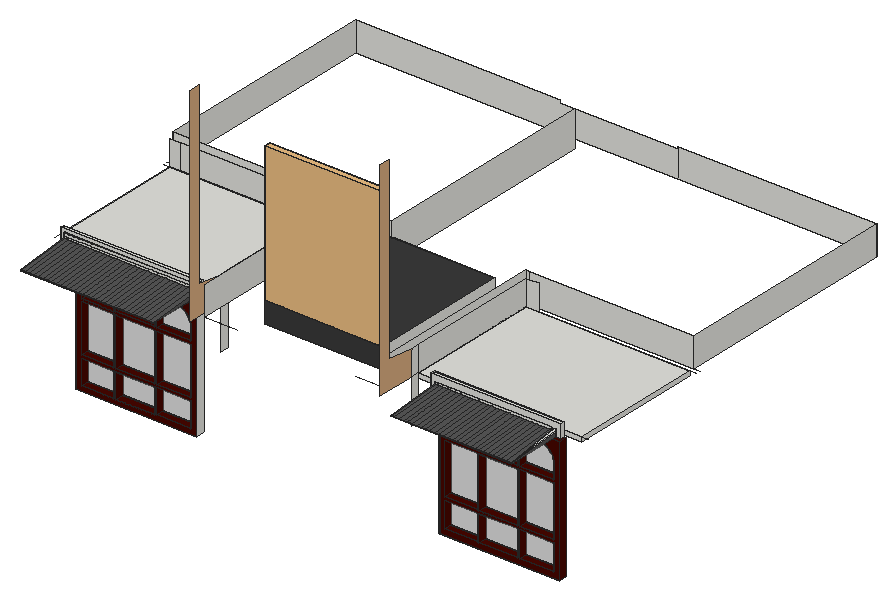
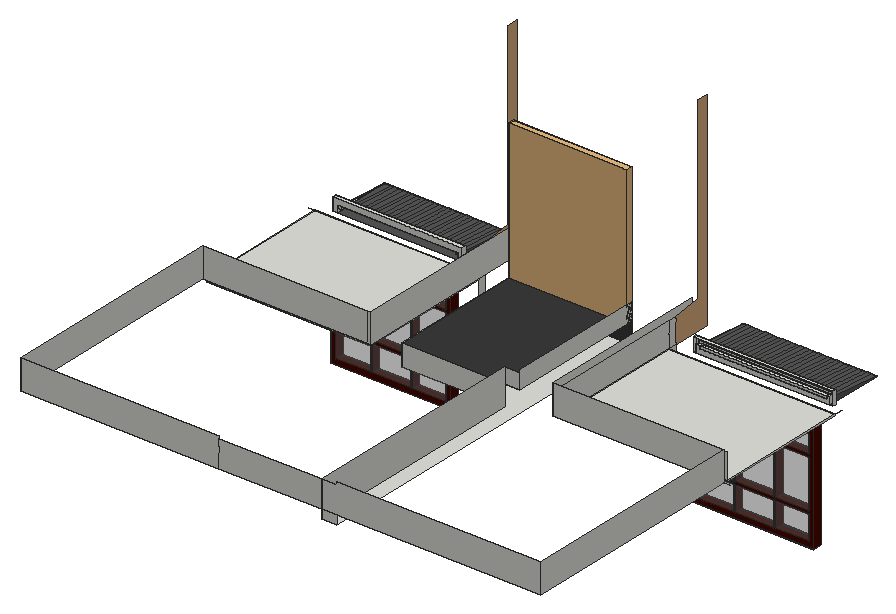
# SketchUp Ruby script. Lengths in inches.
U = 1.inch
M = Sketchup.active_model
def pt(a) = Geom::Point3d.new(a.map { |v| v * U })
def face(e, loops, mat)
  f = e.add_face(loops[0].map { |a| pt(a) })
  loops[1..].each { |l| e.add_face(l.map { |a| pt(a) }).erase! }
  f.material = f.back_material = mat if mat
  f
end
# faces: each face lists its corners as indices into pts; further lists are holes
def faces(e, pts, list, mat = nil) = list.each { |f| face(e, (f[0].is_a?(Array) ? f : [f]).map { |l| l.map { |i| pts[i] } }, mat) }
# xy, xz, yz: faces in a plane at the given z, y or x. An outline is a flat list of corners, or four numbers for a rectangle; further outlines are holes
def ring(l) = l.size == 4 ? [[l[0], l[1]], [l[2], l[1]], [l[2], l[3]], [l[0], l[3]]] : l.each_slice(2).to_a
def flat(e, list, mat, &to3) = list.each { |f| face(e, (f[0].is_a?(Array) ? f : [f]).map { |l| ring(l).map { |u, v| to3.(u, v) } }, mat) }
def xy(e, z, list, mat = nil) = flat(e, list, mat) { |x, y| [x, y, z] }
def xz(e, y, list, mat = nil) = flat(e, list, mat) { |x, z| [x, y, z] }
def yz(e, x, list, mat = nil) = flat(e, list, mat) { |y, z| [x, y, z] }
def lines(e, pts, list) = list.each { |a, b| e.add_line(pt(pts[a]), pt(pts[b])) }
# prism: a flat outline (further loops are holes) pulled along v
def prism(e, loops, v, mat = nil)
  f = face(e, loops, mat); d = Geom::Vector3d.new(v.map { |x| x * U })
  f.pushpull(f.normal.samedirection?(d) ? d.length : -d.length)
end
def box(e, o, s, mat = nil) = prism(e, [[o, [o[0] + s[0], o[1], o[2]], [o[0] + s[0], o[1] + s[1], o[2]], [o[0], o[1] + s[1], o[2]]]], [0, 0, s[2]], mat)
def at(x, y, z, deg = 0) = Geom::Transformation.translation(pt([x, y, z])) * Geom::Transformation.rotation(ORIGIN, Z_AXIS, deg.degrees)
def axes(o, x, y, z) = Geom::Transformation.new([*x, 0, *y, 0, *z, 0, *pt(o).to_a, 1])
def part(name) = M.definitions.add(name)
# library, detail: a bought-in or finely detailed component or shape, given as its bounding box
def library(name, o, s) = part(name).tap { |d| box(d.entities, o, s) }
def detail(e, o, s) = box(e.add_group.entities, o, s)
def put(e, d, t, mat = nil) = e.add_instance(d, t).tap { |i| i.material = mat if mat }
def group(e, t, mat = nil) = e.add_group.tap { |g| g.transformation = t; g.material = mat if mat }.entities
root = M.entities
M.materials.add("[Color C04]").color = [215, 171, 127]
M.materials.add("[Color C08]").color = [71, 7, 0]
M.materials.add("[Color M06]").color = [86, 86, 86]
M.materials.add("[Color M07]").color = [58, 58, 58]
M.materials.add("[Translucent Glass Gray]").color = [128, 128, 128]
M.materials["[Translucent Glass Gray]"].alpha = 0.5
c1 = part("Group\#1")
xy(c1.entities,0,[[0,0,133.1875,11.375]],"[Color C08]")
xy(c1.entities,6.44,[[6.44,0,42.59,11.375],[44.75,0,86.9,11.375],[89.0625,0,126.75,11.375]],"[Color C08]")
xy(c1.entities,37.85,[[6.44,0,42.59,11.375],[44.75,0,86.9,11.375],[89.0625,0,126.75,11.375]],"[Color C08]")
xy(c1.entities,40.75,[[6.44,0,42.59,11.375],[44.75,0,86.9,11.375],[89.0625,0,126.75,11.375]],"[Color C08]")
xy(c1.entities,101.6,[[6.44,0,42.59,11.375],[44.75,0,86.9,11.375],[89.0625,0,126.75,11.375]],"[Color C08]")
xy(c1.entities,104.5,[[6.44,0,42.59,11.375],[44.75,0,86.9,11.375],[89.0625,0,126.75,11.375]],"[Color C08]")
xy(c1.entities,140.62,[[24.51,0,42.59,11.375],[44.75,0,86.9,11.375],[89.0625,0,107.9,11.375]],"[Color C08]")
xy(c1.entities,147.0625,[[0,0,133.1875,11.375]],"[Color C08]")
xz(c1.entities,0,[[[0,0,133.1875,147.0625],[44.75,40.75,86.9,101.6],[89.0625,40.75,126.75,101.6],[6.44,40.75,42.59,101.6],[44.75,104.5,86.9,140.62],[44.75,6.44,86.9,37.85],[89.0625,104.5,89.0625,140.62,107.9,140.62,110.36,140.46,112.78,139.98,115.11,139.1875,117.33,138.1,119.375,136.73,121.23,135.1,122.85,133.25,124.22,131.2,125.3125,128.99,126.1,126.66,126.58,124.24,126.75,121.78,126.75,104.5],[6.44,104.5,6.44,127.03,6.65,127.83,7.8,130.52,9.36,133,11.29,135.21,13.53,137.09,16.03,138.61,18.75,139.72,21.59,140.39,24.51,140.62,42.59,140.62,42.59,104.5],[89.0625,6.44,126.75,37.85],[6.44,6.44,42.59,37.85]]],"[Color C08]")
xz(c1.entities,11.375,[[[0,0,133.1875,147.0625],[44.75,40.75,86.9,101.6],[89.0625,40.75,126.75,101.6],[6.44,40.75,42.59,101.6],[44.75,104.5,86.9,140.62],[44.75,6.44,86.9,37.85],[89.0625,104.5,126.75,104.5,126.75,121.78,126.58,124.24,126.1,126.66,125.3125,128.99,124.22,131.2,122.85,133.25,121.23,135.1,119.375,136.73,117.33,138.1,115.11,139.1875,112.78,139.98,110.36,140.46,107.9,140.62,89.0625,140.62],[6.44,104.5,42.59,104.5,42.59,140.62,24.51,140.62,21.59,140.39,18.75,139.72,16.03,138.61,13.53,137.09,11.29,135.21,9.36,133,7.8,130.52,6.65,127.83,6.44,127.03],[89.0625,6.44,126.75,37.85],[6.44,6.44,42.59,37.85]]],"[Color C08]")
xz(c1.entities,11.375,[[6.44,6.44,42.59,37.85],[44.75,6.44,86.9,37.85],[89.0625,6.44,126.75,37.85],[6.44,40.75,42.59,101.6],[44.75,40.75,86.9,101.6],
  [89.0625,40.75,126.75,101.6],[6.44,104.5,42.59,104.5,42.59,140.62,24.51,140.62,21.59,140.39,18.75,139.72,16.03,138.61,13.53,137.09,11.29,135.21,9.36,133,7.8,130.52,6.65,127.83,6.44,127.03],[44.75,104.5,86.9,140.62],[89.0625,104.5,126.75,104.5,126.75,121.78,126.58,124.24,126.1,126.66,125.3125,128.99,124.22,131.2,122.85,133.25,121.23,135.1,119.375,136.73,117.33,138.1,115.11,139.1875,112.78,139.98,110.36,140.46,107.9,140.62,89.0625,140.62]],"[Translucent Glass Gray]")
yz(c1.entities,0,[[0,0,11.375,147.0625]],"[Color C08]")
yz(c1.entities,6.44,[[0,6.44,11.375,37.85],[0,40.75,11.375,101.6],[0,104.5,11.375,127.03]],"[Color C08]")
yz(c1.entities,42.59,[[0,6.44,11.375,37.85],[0,40.75,11.375,101.6],[0,104.5,11.375,140.62]],"[Color C08]")
yz(c1.entities,44.75,[[0,6.44,11.375,37.85],[0,40.75,11.375,101.6],[0,104.5,11.375,140.62]],"[Color C08]")
yz(c1.entities,86.9,[[0,6.44,11.375,37.85],[0,40.75,11.375,101.6],[0,104.5,11.375,140.62]],"[Color C08]")
yz(c1.entities,89.0625,[[0,6.44,11.375,37.85],[0,40.75,11.375,101.6],[0,104.5,11.375,140.62]],"[Color C08]")
yz(c1.entities,126.75,[[0,6.44,11.375,37.85],[0,40.75,11.375,101.6],[0,104.5,11.375,121.78]],"[Color C08]")
yz(c1.entities,133.1875,[[0,0,11.375,147.0625]],"[Color C08]")
p = [[126.58,11.375,124.24],[126.75,11.375,121.78],[126.75,0,121.78],[126.58,0,124.24],[126.1,11.375,126.66],[126.1,0,126.66],
  [125.3125,11.375,128.99],[125.3125,0,128.99],[6.44,11.375,127.03],[6.65,11.375,127.83],[6.65,0,127.83],[6.44,0,127.03],
  [7.8,11.375,130.52],[7.8,0,130.52],[124.22,11.375,131.2],[124.22,0,131.2],[9.36,11.375,133],[9.36,0,133],
  [122.85,11.375,133.25],[122.85,0,133.25],[11.29,11.375,135.21],[11.29,0,135.21],[121.23,11.375,135.1],[121.23,0,135.1],
  [119.375,11.375,136.73],[119.375,0,136.73],[13.53,11.375,137.09],[13.53,0,137.09],[117.33,11.375,138.1],[117.33,0,138.1],
  [16.03,11.375,138.61],[16.03,0,138.61],[115.11,11.375,139.1875],[115.11,0,139.1875],[18.75,11.375,139.72],[18.75,0,139.72],
  [112.78,11.375,139.98],[112.78,0,139.98],[21.59,11.375,140.39],[21.59,0,140.39],[110.36,11.375,140.46],[110.36,0,140.46],
  [24.51,11.375,140.62],[24.51,0,140.62],[107.9,11.375,140.62],[107.9,0,140.62]]
faces(c1.entities,p,[[0,1,2,3],[4,0,3,5],[6,4,5,7],[8,9,10,11],[9,12,13,10],[14,6,7,15],[12,16,17,13],[18,14,15,19],
  [16,20,21,17],[22,18,19,23],[24,22,23,25],[20,26,27,21],[28,24,25,29],[26,30,31,27],[32,28,29,33],[30,34,35,31],
  [36,32,33,37],[34,38,39,35],[40,36,37,41],[38,42,43,39],[44,40,41,45]],"[Color C08]")
c2 = library("Group\#2",[0,0,0],[72,4.0625,96])
xy(root,60.79,[[546.77,627.4375,708.59,638.0625]])
xy(root,63.5625,[[57.38,626.0625,219.82,638.0625]])
xy(root,221.625,[[57.38,626.0625,219.82,638.0625]])
xy(root,224.25,[[303.29,636.875,303.29,1134.4375,323.73,1134.4375,323.73,826.22,462.79,826.22,462.79,636.875]])
xy(root,227.85,[[546.77,627.4375,708.59,638.0625]])
xy(root,231,[[509.3125,638.0625,730.375,820.1875]])
xy(root,235,[[28.375,638.0625,252.9375,820.1875]])
xy(root,237,[[40.76,621.9375,45.125,626.0625],[225.1875,621.9375,228.51,626.0625],[539.72,621.9375,545.41,627.4375],[708.06,621.9375,714.84,627.4375],[28.375,638.0625,252.9375,820.1875],
  [509.3125,638.0625,730.375,820.1875]])
xy(root,237,[[45.125,547.4375,225.1875,626.0625],[545.41,547.4375,708.06,627.4375]],"[Color M06]")
xy(root,243.26,[[545.41,621.9375,548.77,627.4375]])
xy(root,243.75,[[48.93,621.9375,219.99,626.0625]])
xy(root,244.125,[[219.99,620.875,219.99,621.9375,48.93,621.9375,55,621.9,64,621.84]])
xy(root,246.3125,[[545.41,621.9375,548.77,627.4375],[548.77,621.9375,702.25,627.4375],[702.25,621.9375,708.06,627.4375]])
xy(root,247.25,[[45.125,620.875,48.93,626.0625],[48.93,620.875,219.99,621.9375],[219.99,620.875,225.1875,626.0625],[48.93,621.9375,219.99,626.0625]])
xy(root,251,[[45.125,620.875,225.1875,621.9375]])
xy(root,252.9375,[[303.29,636.875,462.79,826.22]],"[Color M07]")
xy(root,254.125,[[539.72,621.9375,714.84,627.4375]])
xy(root,255.5,[[40.76,621.9375,228.51,626.0625]])
xz(root,547.4375,[[45.125,237,225.1875,237.93],[545.41,237,708.06,237.6875]])
xz(root,620.875,[[45.125,244.125,225.1875,247.25],[45.125,247.25,225.1875,251]])
xz(root,621.9375,[[40.76,237,45.125,237,45.125,251,225.1875,251,225.1875,237,228.51,237,228.51,255.5,40.76,255.5],[539.72,237,545.41,237,545.41,246.3125,708.06,246.3125,708.06,237,714.84,237,714.84,254.125,539.72,254.125],[548.77,243.26,702.25,246.3125],[48.93,243.75,219.99,244.125],[48.93,244.125,219.99,247.25]])
xz(root,626.0625,[[45.125,237,45.125,247.25,48.93,247.25,48.93,243.75,219.99,243.75,219.99,247.25,225.1875,247.25,225.1875,237],[48.93,243.75,219.99,247.25]])
xz(root,627.4375,[[539.72,237,539.72,254.125,714.84,254.125,714.84,237,708.06,237,708.06,246.3125,545.41,246.3125,545.41,237],[545.41,243.26,548.77,246.3125],[702.25,243.26,708.06,246.3125]])
xz(root,636.875,[[303.29,224.25,462.79,252.9375]],"[Color M07]")
xz(root,638.0625,[[509.3125,231,730.375,237],[28.375,235,252.9375,237]])
xz(root,820.1875,[[509.3125,231,526.3125,237],[526.3125,231,730.375,237],[28.375,235,42.875,237],[42.875,235,252.9375,237],[28.375,237,42.875,271.1875],
  [42.875,237,252.9375,271.1875],[509.3125,237,526.3125,271.1875]])
xz(root,826.1875,[[28.375,237,258.9375,276.1875],[509.3125,237,730.375,276.1875]])
xz(root,826.22,[[323.73,224.25,462.79,252.9375],[303.29,252.9375,323.73,273.1875]])
xz(root,1134.4375,[[303.29,224.25,323.73,237],[28.375,237,323.73,237,323.73,273.1875,303.29,273.1875,303.29,276.1875,28.375,276.1875],[323.73,237,462.79,273.1875],[462.79,237,730.375,276.1875]])
yz(root,28.375,[[638.0625,235,820.1875,237],[826.1875,237,1134.4375,276.1875]])
yz(root,40.76,[[621.9375,237,626.0625,255.5]])
yz(root,45.125,[[621.9375,237,626.0625,247.25],[620.875,247.25,621.9375,251]])
yz(root,45.125,[[547.4375,237,547.4375,237.93,620.875,244.125,620.875,247.25,621.9375,247.25,621.9375,237]],"[Color M06]")
yz(root,48.93,[[621.9375,243.75,626.0625,247.25]])
yz(root,57.38,[[626.0625,63.5625,638.0625,221.625]])
yz(root,219.82,[[626.0625,63.5625,638.0625,221.625]])
yz(root,219.99,[[621.9375,243.75,626.0625,247.25]])
yz(root,225.1875,[[621.9375,237,626.0625,247.25],[620.875,247.25,621.9375,251]])
yz(root,225.1875,[[547.4375,237,621.9375,237,621.9375,247.25,620.875,247.25,620.875,244.125,547.4375,237.93]],"[Color M06]")
yz(root,228.51,[[621.9375,237,626.0625,255.5]])
yz(root,252.9375,[[626.0625,177,638.0625,237],[638.0625,235,820.1875,237],[626.0625,237,638.0625,271.1875],[638.0625,237,820.1875,271.1875]])
yz(root,252.9375,[[573.625,237,573.625,516.1875,588.625,516.1875,588.625,275.59,626.0625,271.1875,626.0625,237]],"[Color C04]")
yz(root,258.9375,[[590.9375,237,826.1875,276.1875]])
yz(root,303.29,[[636.875,252.9375,826.22,276.1875]])
yz(root,323.73,[[826.22,224.25,1134.4375,273.1875]])
yz(root,462.79,[[636.875,224.25,826.22,237],[636.875,237,826.22,252.9375]])
yz(root,503.3125,[[590.9375,237,826.375,276.1875]])
yz(root,509.3125,[[627.4375,177,638.0625,237],[638.0625,231,820.1875,237],[627.4375,237,638.0625,271.1875],[638.0625,237,820.1875,271.1875]])
yz(root,509.3125,[[573.625,237,627.4375,237,627.4375,271.1875,588.625,275.59,588.625,516.1875,573.625,516.1875]],"[Color C04]")
yz(root,539.72,[[621.9375,237,627.4375,254.125]])
yz(root,545.41,[[621.9375,237,627.4375,243.26],[621.9375,243.26,627.4375,246.3125]])
yz(root,545.41,[[547.4375,237,547.4375,237.6875,621.9375,243.26,621.9375,237]],"[Color M06]")
yz(root,546.77,[[627.4375,60.79,638.0625,227.85]])
yz(root,548.77,[[621.9375,243.26,627.4375,246.3125]])
yz(root,702.25,[[621.9375,243.26,627.4375,246.3125]])
yz(root,708.06,[[621.9375,237,621.9375,242.875,627.4375,243.26,627.4375,237],[547.4375,237.6875,621.9375,242.875,621.9375,243.26],[621.9375,242.875,627.4375,243.26,621.9375,243.26],[621.9375,243.26,627.4375,246.3125]])
yz(root,708.06,[[547.4375,237,621.9375,237,621.9375,242.875,547.4375,237.6875]],"[Color M06]")
yz(root,708.59,[[627.4375,60.79,638.0625,227.85]])
yz(root,714.84,[[621.9375,237,627.4375,254.125]])
yz(root,730.375,[[638.0625,231,820.1875,237],[826.1875,237,1134.4375,276.1875]])
p = [[509.3125,826.1875,237],[503.3125,826.375,237],[503.3125,826.375,276.1875],[509.3125,826.1875,276.1875],[545.41,547.4375,237.6875],[550.87,547.4375,237.6875],
  [550.87,621.9375,243.26],[548.77,621.9375,243.26],[545.41,621.9375,243.26],[556.37,547.4375,237.6875],[556.37,621.9375,243.26],[562.25,547.4375,237.6875],
  [562.25,621.9375,243.26],[568.25,547.4375,237.6875],[568.25,621.9375,243.26],[574.25,547.4375,237.6875],[574.25,621.9375,243.26],[580.25,547.4375,237.6875],
  [580.25,621.9375,243.26],[586.25,547.4375,237.6875],[586.25,621.9375,243.26],[592.25,547.4375,237.6875],[592.25,621.9375,243.26],[598.25,547.4375,237.6875],
  [598.25,621.9375,243.26],[604.25,547.4375,237.6875],[604.25,621.9375,243.26],[610.25,547.4375,237.6875],[610.25,621.9375,243.26],[616.25,547.4375,237.6875],
  [616.25,621.9375,243.26],[622.25,547.4375,237.6875],[622.25,621.9375,243.26],[628.25,547.4375,237.6875],[628.25,621.9375,243.26],[634.25,547.4375,237.6875],
  [634.25,621.9375,243.26],[640.25,547.4375,237.6875],[640.25,621.9375,243.26],[646.25,547.4375,237.6875],[646.25,621.9375,243.26],[652.25,547.4375,237.6875],
  [652.25,621.9375,243.26],[658.25,547.4375,237.6875],[658.25,621.9375,243.26],[664.25,547.4375,237.6875],[664.25,621.9375,243.26],[670.25,547.4375,237.6875],
  [670.25,621.9375,243.26],[676.25,547.4375,237.6875],[676.25,621.9375,243.26],[682.25,547.4375,237.6875],[682.25,621.9375,243.26],[688.25,547.4375,237.6875],
  [688.25,621.9375,243.26],[694.25,547.4375,237.6875],[694.25,621.9375,243.26],[700.25,547.4375,237.6875],[700.25,621.9375,243.26],[702.25,621.9375,243.26],
  [708.06,547.4375,237.6875],[702.25,627.4375,243.26],[708.06,627.4375,243.26],[708.06,621.9375,242.875],[46.19,547.4375,237.93],[50.82,547.4375,237.93],
  [50.93,620.875,244.125],[45.125,620.875,244.125],[45.125,547.4375,237.93],[56.82,547.4375,237.93],[56.93,620.875,244.125],[62.82,547.4375,237.93],
  [62.93,620.875,244.125],[68.82,547.4375,237.93],[68.93,620.875,244.125],[74.82,547.4375,237.93],[74.93,620.875,244.125],[80.82,547.4375,237.93],
  [80.93,620.875,244.125],[86.82,547.4375,237.93],[86.93,620.875,244.125],[92.82,547.4375,237.93],[92.93,620.875,244.125],[98.82,547.4375,237.93],
  [98.93,620.875,244.125],[104.82,547.4375,237.93],[104.93,620.875,244.125],[110.82,547.4375,237.93],[110.93,620.875,244.125],[116.82,547.4375,237.93],
  [116.93,620.875,244.125],[122.82,547.4375,237.93],[122.93,620.875,244.125],[128.82,547.4375,237.93],[128.93,620.875,244.125],[134.82,547.4375,237.93],
  [134.93,620.875,244.125],[140.82,547.4375,237.93],[140.93,620.875,244.125],[147.01,547.4375,237.93],[147.11,620.875,244.125],[152.82,547.4375,237.93],
  [152.93,620.875,244.125],[158.82,547.4375,237.93],[158.93,620.875,244.125],[164.82,547.4375,237.93],[164.93,620.875,244.125],[170.82,547.4375,237.93],
  [170.93,620.875,244.125],[176.82,547.4375,237.93],[176.93,620.875,244.125],[182.82,547.4375,237.93],[182.93,620.875,244.125],[188.82,547.4375,237.93],
  [188.93,620.875,244.125],[194.82,547.4375,237.93],[194.93,620.875,244.125],[200.82,547.4375,237.93],[200.93,620.875,244.125],[206.82,547.4375,237.93],
  [206.93,620.875,244.125],[212.82,547.4375,237.93],[212.93,620.875,244.125],[218.82,547.4375,237.93],[218.93,620.875,244.125],[219.99,620.875,244.125],
  [225.1875,547.4375,237.93],[225.1875,620.875,244.125],[28.375,826.1875,237],[19.375,826.1875,237],[730.375,826.1875,237],[739.375,826.1875,237],
  [28.375,820.1875,237],[19.375,820.1875,237],[28.375,638.0625,237],[28.375,626.0625,237],[730.375,820.1875,237],[739.375,820.1875,237],
  [730.375,638.0625,237],[739.375,638.0625,237],[258.9375,590.9375,237],[303.29,590.9375,237],[462.79,590.9375,237],[503.3125,590.9375,237]]
faces(root,p,[[0,1,2,3],[61,59,60],[62,61,60,63]])
faces(root,p,[[4,5,6,7,8],[5,9,10,6],[9,11,12,10],[11,13,14,12],[13,15,16,14],[15,17,18,16],[17,19,20,18],[19,21,22,20],
  [21,23,24,22],[23,25,26,24],[25,27,28,26],[27,29,30,28],[29,31,32,30],[31,33,34,32],[33,35,36,34],[35,37,38,36],
  [37,39,40,38],[39,41,42,40],[41,43,44,42],[43,45,46,44],[45,47,48,46],[47,49,50,48],[49,51,52,50],[51,53,54,52],
  [53,55,56,54],[55,57,58,56],[59,58,57,60],[64,65,66,67,68],[65,69,70,66],[69,71,72,70],[71,73,74,72],[73,75,76,74],
  [75,77,78,76],[77,79,80,78],[79,81,82,80],[81,83,84,82],[83,85,86,84],[85,87,88,86],[87,89,90,88],[89,91,92,90],
  [91,93,94,92],[93,95,96,94],[95,97,98,96],[97,99,100,98],[99,101,102,100],[101,103,104,102],[103,105,106,104],[105,107,108,106],
  [107,109,110,108],[109,111,112,110],[111,113,114,112],[113,115,116,114],[115,117,118,116],[117,119,120,118],[119,121,122,120],[121,123,124,122],
  [125,124,123,126,127]],"[Color M06]")
lines(root,p,[[128,129],[130,131],[132,133],[134,135],[136,137],[138,139],[140,141],[142,143]])
put(root,c1,axes([545.57,627.4375,60.79],[1.224,0,0],[0,1,0],[0,0,1.136]))
put(root,c1,axes([56.79,626.0625,63.5625],[1.224,0,0],[0,1,0],[0,0,1.0748]))
put(root,c2,axes([303.29,636.875,252.9375],[2.21528,0,0],[0,2.16,0],[0,0,1.9425]))
